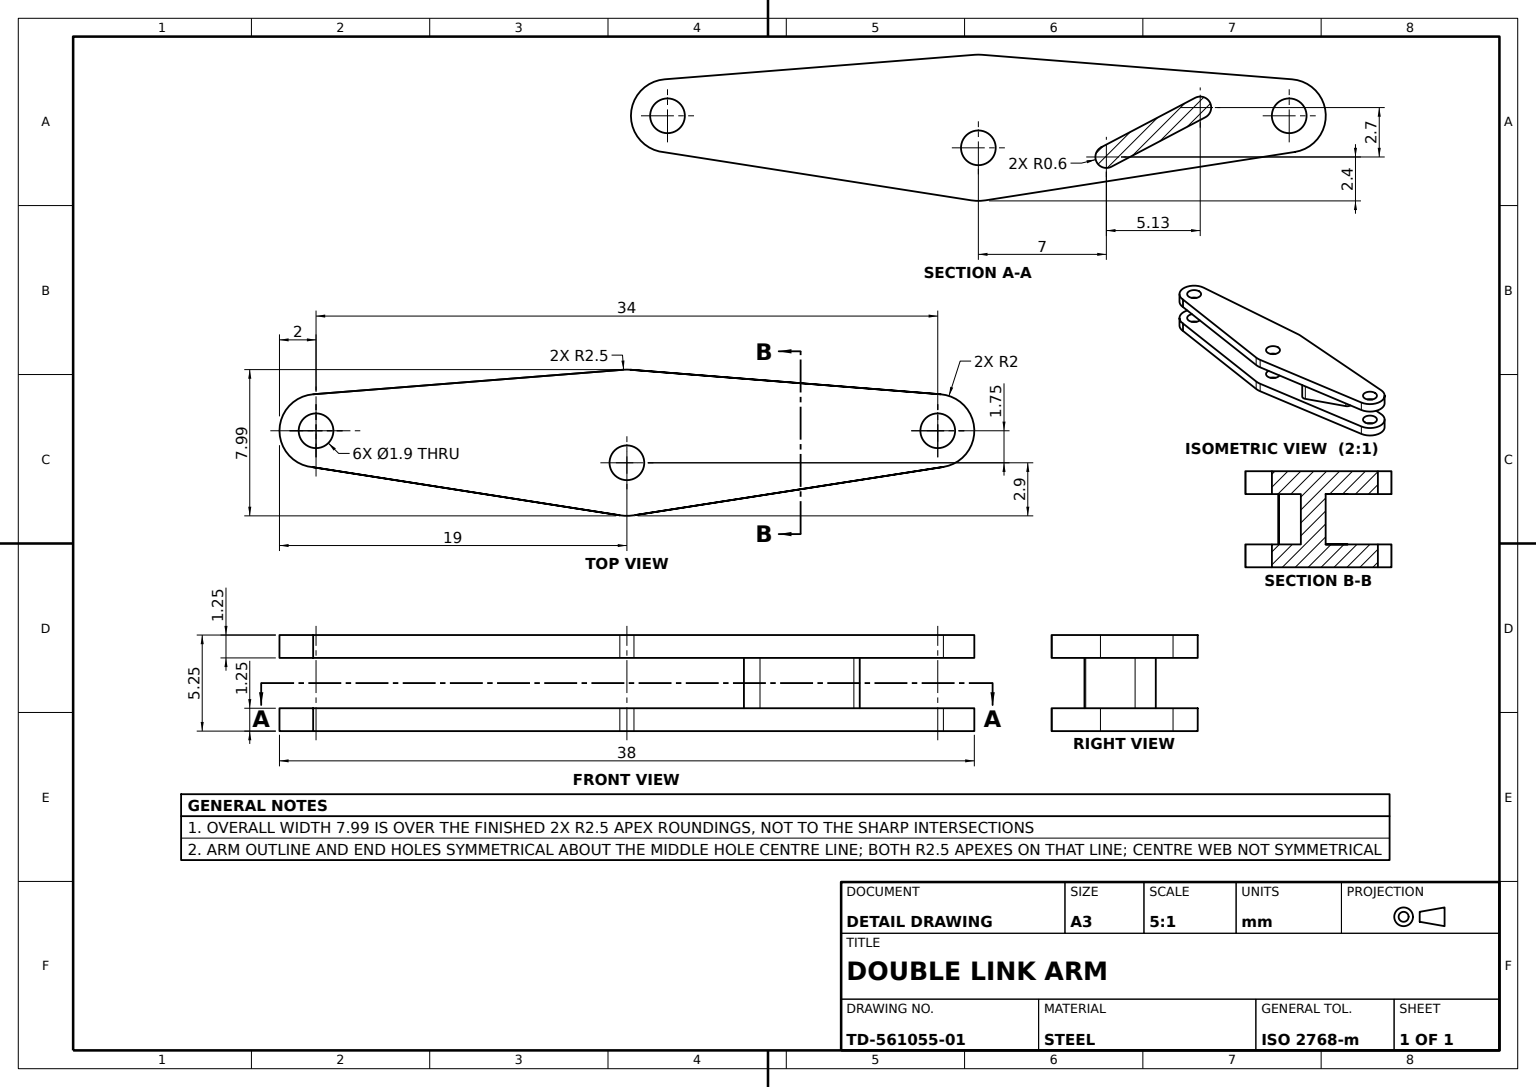
ISO-10303-21;
HEADER;
FILE_DESCRIPTION((''),'2;1');
FILE_NAME('','',(''),(''),'','','');
FILE_SCHEMA(('AUTOMOTIVE_DESIGN'));
ENDSEC;
DATA;
#1=APPLICATION_CONTEXT('');
#2=PRODUCT_CONTEXT('',#1,'mechanical');
#3=PRODUCT('','','',(#2));
#4=PRODUCT_DEFINITION_FORMATION('','',#3);
#5=PRODUCT_DEFINITION_CONTEXT('',#1,'design');
#6=PRODUCT_DEFINITION('','',#4,#5);
#7=PRODUCT_DEFINITION_SHAPE('','',#6);
#8=(LENGTH_UNIT()NAMED_UNIT(*)SI_UNIT(.MILLI.,.METRE.));
#9=(NAMED_UNIT(*)PLANE_ANGLE_UNIT()SI_UNIT($,.RADIAN.));
#10=(NAMED_UNIT(*)SI_UNIT($,.STERADIAN.)SOLID_ANGLE_UNIT());
#11=UNCERTAINTY_MEASURE_WITH_UNIT(LENGTH_MEASURE(1.E-05),#8,'distance_accuracy_value','');
#12=(GEOMETRIC_REPRESENTATION_CONTEXT(3)GLOBAL_UNCERTAINTY_ASSIGNED_CONTEXT((#11))GLOBAL_UNIT_ASSIGNED_CONTEXT((#8,#9,#10))REPRESENTATION_CONTEXT('',''));
#13=CARTESIAN_POINT('',(7.,-1.375,2.85));
#14=VERTEX_POINT('',#13);
#15=CARTESIAN_POINT('',(7.,1.375,2.85));
#16=VERTEX_POINT('',#15);
#17=CARTESIAN_POINT('',(7.,-2.627,2.85));
#18=DIRECTION('',(0.,1.,0.));
#19=VECTOR('',#18,1000.);
#20=LINE('',#17,#19);
#21=EDGE_CURVE('',#14,#16,#20,.T.);
#22=ORIENTED_EDGE('',*,*,#21,.F.);
#23=CARTESIAN_POINT('',(7.27931,-1.375,2.781023));
#24=VERTEX_POINT('',#23);
#25=CARTESIAN_POINT('',(7.,-1.375,2.25));
#26=DIRECTION('',(0.,0.,-1.));
#27=AXIS2_PLACEMENT_3D('',#25,#18,#26);
#28=CIRCLE('',#27,0.6);
#29=EDGE_CURVE('',#14,#24,#28,.T.);
#30=ORIENTED_EDGE('',*,*,#29,.T.);
#31=CARTESIAN_POINT('',(7.27931,1.375,2.781023));
#32=VERTEX_POINT('',#31);
#33=CARTESIAN_POINT('',(7.27931,-2.627,2.781023));
#34=LINE('',#33,#19);
#35=EDGE_CURVE('',#24,#32,#34,.T.);
#36=ORIENTED_EDGE('',*,*,#35,.T.);
#37=CARTESIAN_POINT('',(7.,1.375,2.25));
#38=DIRECTION('',(0.,0.,1.));
#39=AXIS2_PLACEMENT_3D('',#37,#18,#38);
#40=CIRCLE('',#39,0.6);
#41=EDGE_CURVE('',#16,#32,#40,.T.);
#42=ORIENTED_EDGE('',*,*,#41,.F.);
#43=EDGE_LOOP('',(#22,#30,#36,#42));
#44=FACE_OUTER_BOUND('',#43,.T.);
#45=CARTESIAN_POINT('',(7.,-2.627,2.25));
#46=AXIS2_PLACEMENT_3D('',#45,#18,#38);
#47=CYLINDRICAL_SURFACE('',#46,0.6);
#48=ADVANCED_FACE('',(#44),#47,.T.);
#49=CARTESIAN_POINT('',(-17.,-2.625,-0.95));
#50=VERTEX_POINT('',#49);
#51=CARTESIAN_POINT('',(-17.,-2.625,0.95));
#52=VERTEX_POINT('',#51);
#53=CARTESIAN_POINT('',(-17.,-2.625,0.));
#54=AXIS2_PLACEMENT_3D('',#53,#18,#38);
#55=CIRCLE('',#54,0.95);
#56=EDGE_CURVE('',#50,#52,#55,.T.);
#57=ORIENTED_EDGE('',*,*,#56,.F.);
#58=CARTESIAN_POINT('',(-17.,-1.375,-0.95));
#59=VERTEX_POINT('',#58);
#60=CARTESIAN_POINT('',(-17.,2.625,-0.95));
#61=DIRECTION('',(0.,-1.,0.));
#62=VECTOR('',#61,1000.);
#63=LINE('',#60,#62);
#64=EDGE_CURVE('',#59,#50,#63,.T.);
#65=ORIENTED_EDGE('',*,*,#64,.F.);
#66=CARTESIAN_POINT('',(-17.,-1.375,0.95));
#67=VERTEX_POINT('',#66);
#68=CARTESIAN_POINT('',(-17.,-1.375,0.));
#69=AXIS2_PLACEMENT_3D('',#68,#61,#26);
#70=CIRCLE('',#69,0.95);
#71=EDGE_CURVE('',#67,#59,#70,.T.);
#72=ORIENTED_EDGE('',*,*,#71,.F.);
#73=CARTESIAN_POINT('',(-17.,2.625,0.95));
#74=LINE('',#73,#62);
#75=EDGE_CURVE('',#67,#52,#74,.T.);
#76=ORIENTED_EDGE('',*,*,#75,.T.);
#77=EDGE_LOOP('',(#57,#65,#72,#76));
#78=FACE_OUTER_BOUND('',#77,.T.);
#79=CARTESIAN_POINT('',(-17.,2.625,0.));
#80=AXIS2_PLACEMENT_3D('',#79,#61,#26);
#81=CYLINDRICAL_SURFACE('',#80,0.95);
#82=ADVANCED_FACE('',(#78),#81,.F.);
#83=CARTESIAN_POINT('',(17.,2.625,-0.95));
#84=VERTEX_POINT('',#83);
#85=CARTESIAN_POINT('',(17.,1.375,-0.95));
#86=VERTEX_POINT('',#85);
#87=LINE('',#83,#62);
#88=EDGE_CURVE('',#84,#86,#87,.T.);
#89=ORIENTED_EDGE('',*,*,#88,.T.);
#90=CARTESIAN_POINT('',(17.,1.375,0.95));
#91=VERTEX_POINT('',#90);
#92=CARTESIAN_POINT('',(17.,1.375,0.));
#93=AXIS2_PLACEMENT_3D('',#92,#18,#38);
#94=CIRCLE('',#93,0.95);
#95=EDGE_CURVE('',#91,#86,#94,.T.);
#96=ORIENTED_EDGE('',*,*,#95,.F.);
#97=CARTESIAN_POINT('',(17.,2.625,0.95));
#98=VERTEX_POINT('',#97);
#99=LINE('',#97,#62);
#100=EDGE_CURVE('',#98,#91,#99,.T.);
#101=ORIENTED_EDGE('',*,*,#100,.F.);
#102=CARTESIAN_POINT('',(17.,2.625,0.));
#103=AXIS2_PLACEMENT_3D('',#102,#18,#38);
#104=CIRCLE('',#103,0.95);
#105=EDGE_CURVE('',#98,#84,#104,.T.);
#106=ORIENTED_EDGE('',*,*,#105,.T.);
#107=EDGE_LOOP('',(#89,#96,#101,#106));
#108=FACE_OUTER_BOUND('',#107,.T.);
#109=AXIS2_PLACEMENT_3D('',#102,#61,#26);
#110=CYLINDRICAL_SURFACE('',#109,0.95);
#111=ADVANCED_FACE('',(#108),#110,.F.);
#112=CARTESIAN_POINT('',(17.157598,2.625,-1.993781));
#113=VERTEX_POINT('',#112);
#114=CARTESIAN_POINT('',(17.157598,1.375,-1.993781));
#115=VERTEX_POINT('',#114);
#116=LINE('',#112,#62);
#117=EDGE_CURVE('',#113,#115,#116,.T.);
#118=ORIENTED_EDGE('',*,*,#117,.F.);
#119=CARTESIAN_POINT('',(17.30874,2.625,1.976026));
#120=VERTEX_POINT('',#119);
#121=CIRCLE('',#103,2.);
#122=EDGE_CURVE('',#120,#113,#121,.T.);
#123=ORIENTED_EDGE('',*,*,#122,.F.);
#124=CARTESIAN_POINT('',(17.30874,1.375,1.976026));
#125=VERTEX_POINT('',#124);
#126=LINE('',#119,#62);
#127=EDGE_CURVE('',#120,#125,#126,.T.);
#128=ORIENTED_EDGE('',*,*,#127,.T.);
#129=CIRCLE('',#93,2.);
#130=EDGE_CURVE('',#125,#115,#129,.T.);
#131=ORIENTED_EDGE('',*,*,#130,.T.);
#132=EDGE_LOOP('',(#118,#123,#128,#131));
#133=FACE_OUTER_BOUND('',#132,.T.);
#134=CYLINDRICAL_SURFACE('',#109,2.);
#135=ADVANCED_FACE('',(#133),#134,.T.);
#136=CARTESIAN_POINT('',(-17.157598,2.625,1.993781));
#137=VERTEX_POINT('',#136);
#138=CARTESIAN_POINT('',(-17.157598,1.375,1.993781));
#139=VERTEX_POINT('',#138);
#140=LINE('',#136,#62);
#141=EDGE_CURVE('',#137,#139,#140,.T.);
#142=ORIENTED_EDGE('',*,*,#141,.T.);
#143=CARTESIAN_POINT('',(-0.386332,1.375,4.619904));
#144=VERTEX_POINT('',#143);
#145=DIRECTION('',(0.987961552,0.,0.154699618));
#146=VECTOR('',#145,1000.);
#147=LINE('',#138,#146);
#148=EDGE_CURVE('',#139,#144,#147,.T.);
#149=ORIENTED_EDGE('',*,*,#148,.T.);
#150=CARTESIAN_POINT('',(-0.386332,2.625,4.619904));
#151=VERTEX_POINT('',#150);
#152=LINE('',#150,#62);
#153=EDGE_CURVE('',#151,#144,#152,.T.);
#154=ORIENTED_EDGE('',*,*,#153,.F.);
#155=LINE('',#136,#146);
#156=EDGE_CURVE('',#137,#151,#155,.T.);
#157=ORIENTED_EDGE('',*,*,#156,.F.);
#158=EDGE_LOOP('',(#142,#149,#154,#157));
#159=FACE_OUTER_BOUND('',#158,.T.);
#160=DIRECTION('',(0.154699618,0.,-0.987961552));
#161=DIRECTION('',(-0.987961552,0.,-0.154699618));
#162=AXIS2_PLACEMENT_3D('',#136,#160,#161);
#163=PLANE('',#162);
#164=ADVANCED_FACE('',(#159),#163,.F.);
#165=ORIENTED_EDGE('',*,*,#156,.T.);
#166=CARTESIAN_POINT('',(0.386342,2.625,4.620033));
#167=VERTEX_POINT('',#166);
#168=CARTESIAN_POINT('',(0.000417,2.625,2.15));
#169=AXIS2_PLACEMENT_3D('',#168,#18,#38);
#170=CIRCLE('',#169,2.5);
#171=EDGE_CURVE('',#151,#167,#170,.T.);
#172=ORIENTED_EDGE('',*,*,#171,.T.);
#173=DIRECTION('',(0.988013086,0.,-0.154370148));
#174=VECTOR('',#173,1000.);
#175=LINE('',#166,#174);
#176=EDGE_CURVE('',#167,#120,#175,.T.);
#177=ORIENTED_EDGE('',*,*,#176,.T.);
#178=ORIENTED_EDGE('',*,*,#122,.T.);
#179=CARTESIAN_POINT('',(0.196998,2.625,-3.334428));
#180=VERTEX_POINT('',#179);
#181=DIRECTION('',(-0.996890523,0.,-0.078799015));
#182=VECTOR('',#181,1000.);
#183=LINE('',#179,#182);
#184=EDGE_CURVE('',#113,#180,#183,.T.);
#185=ORIENTED_EDGE('',*,*,#184,.T.);
#186=CARTESIAN_POINT('',(0.,2.625,-3.342202));
#187=VERTEX_POINT('',#186);
#188=CARTESIAN_POINT('',(0.,2.625,-0.842202));
#189=AXIS2_PLACEMENT_3D('',#188,#18,#38);
#190=CIRCLE('',#189,2.5);
#191=EDGE_CURVE('',#180,#187,#190,.T.);
#192=ORIENTED_EDGE('',*,*,#191,.T.);
#193=CARTESIAN_POINT('',(-0.196998,2.625,-3.334428));
#194=VERTEX_POINT('',#193);
#195=EDGE_CURVE('',#187,#194,#190,.T.);
#196=ORIENTED_EDGE('',*,*,#195,.T.);
#197=CARTESIAN_POINT('',(-17.157598,2.625,-1.993781));
#198=VERTEX_POINT('',#197);
#199=DIRECTION('',(-0.996890523,0.,0.078799015));
#200=VECTOR('',#199,1000.);
#201=LINE('',#197,#200);
#202=EDGE_CURVE('',#194,#198,#201,.T.);
#203=ORIENTED_EDGE('',*,*,#202,.T.);
#204=AXIS2_PLACEMENT_3D('',#79,#18,#38);
#205=CIRCLE('',#204,2.);
#206=EDGE_CURVE('',#198,#137,#205,.T.);
#207=ORIENTED_EDGE('',*,*,#206,.T.);
#208=EDGE_LOOP('',(#165,#172,#177,#178,#185,#192,#196,#203,#207));
#209=FACE_OUTER_BOUND('',#208,.T.);
#210=ORIENTED_EDGE('',*,*,#105,.F.);
#211=EDGE_CURVE('',#84,#98,#104,.T.);
#212=ORIENTED_EDGE('',*,*,#211,.F.);
#213=EDGE_LOOP('',(#210,#212));
#214=FACE_BOUND('',#213,.T.);
#215=VERTEX_POINT('',#73);
#216=VERTEX_POINT('',#60);
#217=CIRCLE('',#204,0.95);
#218=EDGE_CURVE('',#215,#216,#217,.T.);
#219=ORIENTED_EDGE('',*,*,#218,.F.);
#220=EDGE_CURVE('',#216,#215,#217,.T.);
#221=ORIENTED_EDGE('',*,*,#220,.F.);
#222=EDGE_LOOP('',(#219,#221));
#223=FACE_BOUND('',#222,.T.);
#224=CARTESIAN_POINT('',(0.,2.625,0.8));
#225=VERTEX_POINT('',#224);
#226=CARTESIAN_POINT('',(0.,2.625,2.7));
#227=VERTEX_POINT('',#226);
#228=CARTESIAN_POINT('',(0.,2.625,1.75));
#229=AXIS2_PLACEMENT_3D('',#228,#18,#38);
#230=CIRCLE('',#229,0.95);
#231=EDGE_CURVE('',#225,#227,#230,.T.);
#232=ORIENTED_EDGE('',*,*,#231,.F.);
#233=EDGE_CURVE('',#227,#225,#230,.T.);
#234=ORIENTED_EDGE('',*,*,#233,.F.);
#235=EDGE_LOOP('',(#232,#234));
#236=FACE_BOUND('',#235,.T.);
#237=PLANE('',#169);
#238=ADVANCED_FACE('',(#209,#214,#223,#236),#237,.T.);
#239=CARTESIAN_POINT('',(11.853915,-1.375,-0.981023));
#240=VERTEX_POINT('',#239);
#241=CARTESIAN_POINT('',(11.853915,1.375,-0.981023));
#242=VERTEX_POINT('',#241);
#243=CARTESIAN_POINT('',(11.853915,-2.627,-0.981023));
#244=LINE('',#243,#19);
#245=EDGE_CURVE('',#240,#242,#244,.T.);
#246=ORIENTED_EDGE('',*,*,#245,.T.);
#247=CARTESIAN_POINT('',(12.412535,1.375,0.081023));
#248=VERTEX_POINT('',#247);
#249=CARTESIAN_POINT('',(12.133225,1.375,-0.45));
#250=AXIS2_PLACEMENT_3D('',#249,#18,#38);
#251=CIRCLE('',#250,0.6);
#252=EDGE_CURVE('',#248,#242,#251,.T.);
#253=ORIENTED_EDGE('',*,*,#252,.F.);
#254=CARTESIAN_POINT('',(12.412535,-1.375,0.081023));
#255=VERTEX_POINT('',#254);
#256=CARTESIAN_POINT('',(12.412535,-2.627,0.081023));
#257=LINE('',#256,#19);
#258=EDGE_CURVE('',#255,#248,#257,.T.);
#259=ORIENTED_EDGE('',*,*,#258,.F.);
#260=CARTESIAN_POINT('',(12.133225,-1.375,-0.45));
#261=AXIS2_PLACEMENT_3D('',#260,#18,#26);
#262=CIRCLE('',#261,0.6);
#263=EDGE_CURVE('',#255,#240,#262,.T.);
#264=ORIENTED_EDGE('',*,*,#263,.T.);
#265=EDGE_LOOP('',(#246,#253,#259,#264));
#266=FACE_OUTER_BOUND('',#265,.T.);
#267=CARTESIAN_POINT('',(12.133225,-2.627,-0.45));
#268=AXIS2_PLACEMENT_3D('',#267,#18,#38);
#269=CYLINDRICAL_SURFACE('',#268,0.6);
#270=ADVANCED_FACE('',(#266),#269,.T.);
#271=CARTESIAN_POINT('',(0.386342,-1.375,4.620033));
#272=VERTEX_POINT('',#271);
#273=CARTESIAN_POINT('',(0.386342,-2.625,4.620033));
#274=VERTEX_POINT('',#273);
#275=LINE('',#166,#62);
#276=EDGE_CURVE('',#272,#274,#275,.T.);
#277=ORIENTED_EDGE('',*,*,#276,.T.);
#278=CARTESIAN_POINT('',(17.30874,-2.625,1.976026));
#279=VERTEX_POINT('',#278);
#280=LINE('',#273,#174);
#281=EDGE_CURVE('',#274,#279,#280,.T.);
#282=ORIENTED_EDGE('',*,*,#281,.T.);
#283=CARTESIAN_POINT('',(17.30874,-1.375,1.976026));
#284=VERTEX_POINT('',#283);
#285=EDGE_CURVE('',#284,#279,#126,.T.);
#286=ORIENTED_EDGE('',*,*,#285,.F.);
#287=DIRECTION('',(-0.988013086,0.,0.154370148));
#288=VECTOR('',#287,1000.);
#289=LINE('',#271,#288);
#290=EDGE_CURVE('',#284,#272,#289,.T.);
#291=ORIENTED_EDGE('',*,*,#290,.T.);
#292=EDGE_LOOP('',(#277,#282,#286,#291));
#293=FACE_OUTER_BOUND('',#292,.T.);
#294=DIRECTION('',(-0.154370148,0.,-0.988013086));
#295=AXIS2_PLACEMENT_3D('',#166,#294,#287);
#296=PLANE('',#295);
#297=ADVANCED_FACE('',(#293),#296,.F.);
#298=CARTESIAN_POINT('',(0.,1.375,2.7));
#299=VERTEX_POINT('',#298);
#300=LINE('',#226,#62);
#301=EDGE_CURVE('',#227,#299,#300,.T.);
#302=ORIENTED_EDGE('',*,*,#301,.T.);
#303=CARTESIAN_POINT('',(0.,1.375,0.8));
#304=VERTEX_POINT('',#303);
#305=CARTESIAN_POINT('',(0.,1.375,1.75));
#306=AXIS2_PLACEMENT_3D('',#305,#18,#38);
#307=CIRCLE('',#306,0.95);
#308=EDGE_CURVE('',#304,#299,#307,.T.);
#309=ORIENTED_EDGE('',*,*,#308,.F.);
#310=LINE('',#224,#62);
#311=EDGE_CURVE('',#225,#304,#310,.T.);
#312=ORIENTED_EDGE('',*,*,#311,.F.);
#313=ORIENTED_EDGE('',*,*,#231,.T.);
#314=EDGE_LOOP('',(#302,#309,#312,#313));
#315=FACE_OUTER_BOUND('',#314,.T.);
#316=AXIS2_PLACEMENT_3D('',#228,#61,#26);
#317=CYLINDRICAL_SURFACE('',#316,0.95);
#318=ADVANCED_FACE('',(#315),#317,.F.);
#319=EDGE_CURVE('',#59,#67,#70,.T.);
#320=ORIENTED_EDGE('',*,*,#319,.T.);
#321=ORIENTED_EDGE('',*,*,#71,.T.);
#322=EDGE_LOOP('',(#320,#321));
#323=FACE_BOUND('',#322,.T.);
#324=CARTESIAN_POINT('',(17.,-1.375,0.95));
#325=VERTEX_POINT('',#324);
#326=CARTESIAN_POINT('',(17.,-1.375,-0.95));
#327=VERTEX_POINT('',#326);
#328=CARTESIAN_POINT('',(17.,-1.375,0.));
#329=AXIS2_PLACEMENT_3D('',#328,#61,#26);
#330=CIRCLE('',#329,0.95);
#331=EDGE_CURVE('',#325,#327,#330,.T.);
#332=ORIENTED_EDGE('',*,*,#331,.T.);
#333=EDGE_CURVE('',#327,#325,#330,.T.);
#334=ORIENTED_EDGE('',*,*,#333,.T.);
#335=EDGE_LOOP('',(#332,#334));
#336=FACE_BOUND('',#335,.T.);
#337=CARTESIAN_POINT('',(-0.196998,-1.375,-3.334428));
#338=VERTEX_POINT('',#337);
#339=CARTESIAN_POINT('',(0.,-1.375,-3.342202));
#340=VERTEX_POINT('',#339);
#341=CARTESIAN_POINT('',(0.,-1.375,-0.842202));
#342=AXIS2_PLACEMENT_3D('',#341,#61,#26);
#343=CIRCLE('',#342,2.5);
#344=EDGE_CURVE('',#338,#340,#343,.T.);
#345=ORIENTED_EDGE('',*,*,#344,.F.);
#346=CARTESIAN_POINT('',(-17.157598,-1.375,-1.993781));
#347=VERTEX_POINT('',#346);
#348=DIRECTION('',(0.996890523,0.,-0.078799015));
#349=VECTOR('',#348,1000.);
#350=LINE('',#346,#349);
#351=EDGE_CURVE('',#347,#338,#350,.T.);
#352=ORIENTED_EDGE('',*,*,#351,.F.);
#353=CARTESIAN_POINT('',(-17.157598,-1.375,1.993781));
#354=VERTEX_POINT('',#353);
#355=CIRCLE('',#69,2.);
#356=EDGE_CURVE('',#354,#347,#355,.T.);
#357=ORIENTED_EDGE('',*,*,#356,.F.);
#358=CARTESIAN_POINT('',(-0.386332,-1.375,4.619904));
#359=VERTEX_POINT('',#358);
#360=VECTOR('',#161,1000.);
#361=LINE('',#353,#360);
#362=EDGE_CURVE('',#359,#354,#361,.T.);
#363=ORIENTED_EDGE('',*,*,#362,.F.);
#364=CARTESIAN_POINT('',(0.000417,-1.375,2.15));
#365=AXIS2_PLACEMENT_3D('',#364,#61,#26);
#366=CIRCLE('',#365,2.5);
#367=EDGE_CURVE('',#272,#359,#366,.T.);
#368=ORIENTED_EDGE('',*,*,#367,.F.);
#369=ORIENTED_EDGE('',*,*,#290,.F.);
#370=CARTESIAN_POINT('',(17.157598,-1.375,-1.993781));
#371=VERTEX_POINT('',#370);
#372=CIRCLE('',#329,2.);
#373=EDGE_CURVE('',#371,#284,#372,.T.);
#374=ORIENTED_EDGE('',*,*,#373,.F.);
#375=CARTESIAN_POINT('',(0.196998,-1.375,-3.334428));
#376=VERTEX_POINT('',#375);
#377=DIRECTION('',(0.996890523,0.,0.078799015));
#378=VECTOR('',#377,1000.);
#379=LINE('',#375,#378);
#380=EDGE_CURVE('',#376,#371,#379,.T.);
#381=ORIENTED_EDGE('',*,*,#380,.F.);
#382=EDGE_CURVE('',#340,#376,#343,.T.);
#383=ORIENTED_EDGE('',*,*,#382,.F.);
#384=EDGE_LOOP('',(#345,#352,#357,#363,#368,#369,#374,#381,#383));
#385=FACE_OUTER_BOUND('',#384,.T.);
#386=DIRECTION('',(0.885038812,0.,-0.465517241));
#387=VECTOR('',#386,1000.);
#388=LINE('',#23,#387);
#389=EDGE_CURVE('',#24,#255,#388,.T.);
#390=ORIENTED_EDGE('',*,*,#389,.F.);
#391=ORIENTED_EDGE('',*,*,#29,.F.);
#392=CARTESIAN_POINT('',(6.72069,-1.375,1.718977));
#393=VERTEX_POINT('',#392);
#394=EDGE_CURVE('',#393,#14,#28,.T.);
#395=ORIENTED_EDGE('',*,*,#394,.F.);
#396=DIRECTION('',(-0.885038812,0.,0.465517241));
#397=VECTOR('',#396,1000.);
#398=LINE('',#392,#397);
#399=EDGE_CURVE('',#240,#393,#398,.T.);
#400=ORIENTED_EDGE('',*,*,#399,.F.);
#401=ORIENTED_EDGE('',*,*,#263,.F.);
#402=EDGE_LOOP('',(#390,#391,#395,#400,#401));
#403=FACE_BOUND('',#402,.T.);
#404=CARTESIAN_POINT('',(0.,-1.375,2.7));
#405=VERTEX_POINT('',#404);
#406=CARTESIAN_POINT('',(0.,-1.375,0.8));
#407=VERTEX_POINT('',#406);
#408=CARTESIAN_POINT('',(0.,-1.375,1.75));
#409=AXIS2_PLACEMENT_3D('',#408,#61,#26);
#410=CIRCLE('',#409,0.95);
#411=EDGE_CURVE('',#405,#407,#410,.T.);
#412=ORIENTED_EDGE('',*,*,#411,.T.);
#413=EDGE_CURVE('',#407,#405,#410,.T.);
#414=ORIENTED_EDGE('',*,*,#413,.T.);
#415=EDGE_LOOP('',(#412,#414));
#416=FACE_BOUND('',#415,.T.);
#417=CARTESIAN_POINT('',(-19.564242,-1.375,-22.625));
#418=AXIS2_PLACEMENT_3D('',#417,#61,#26);
#419=PLANE('',#418);
#420=ADVANCED_FACE('',(#323,#336,#385,#403,#416),#419,.F.);
#421=ORIENTED_EDGE('',*,*,#258,.T.);
#422=LINE('',#31,#387);
#423=EDGE_CURVE('',#32,#248,#422,.T.);
#424=ORIENTED_EDGE('',*,*,#423,.F.);
#425=ORIENTED_EDGE('',*,*,#35,.F.);
#426=ORIENTED_EDGE('',*,*,#389,.T.);
#427=EDGE_LOOP('',(#421,#424,#425,#426));
#428=FACE_OUTER_BOUND('',#427,.T.);
#429=DIRECTION('',(0.465517241,0.,0.885038812));
#430=AXIS2_PLACEMENT_3D('',#33,#429,#386);
#431=PLANE('',#430);
#432=ADVANCED_FACE('',(#428),#431,.T.);
#433=ORIENTED_EDGE('',*,*,#380,.T.);
#434=CARTESIAN_POINT('',(17.157598,-2.625,-1.993781));
#435=VERTEX_POINT('',#434);
#436=EDGE_CURVE('',#371,#435,#116,.T.);
#437=ORIENTED_EDGE('',*,*,#436,.T.);
#438=CARTESIAN_POINT('',(0.196998,-2.625,-3.334428));
#439=VERTEX_POINT('',#438);
#440=LINE('',#438,#182);
#441=EDGE_CURVE('',#435,#439,#440,.T.);
#442=ORIENTED_EDGE('',*,*,#441,.T.);
#443=LINE('',#179,#62);
#444=EDGE_CURVE('',#376,#439,#443,.T.);
#445=ORIENTED_EDGE('',*,*,#444,.F.);
#446=EDGE_LOOP('',(#433,#437,#442,#445));
#447=FACE_OUTER_BOUND('',#446,.T.);
#448=DIRECTION('',(-0.078799015,0.,0.996890523));
#449=AXIS2_PLACEMENT_3D('',#179,#448,#377);
#450=PLANE('',#449);
#451=ADVANCED_FACE('',(#447),#450,.F.);
#452=ORIENTED_EDGE('',*,*,#276,.F.);
#453=ORIENTED_EDGE('',*,*,#367,.T.);
#454=CARTESIAN_POINT('',(-0.386332,-2.625,4.619904));
#455=VERTEX_POINT('',#454);
#456=EDGE_CURVE('',#359,#455,#152,.T.);
#457=ORIENTED_EDGE('',*,*,#456,.T.);
#458=CARTESIAN_POINT('',(0.000417,-2.625,2.15));
#459=AXIS2_PLACEMENT_3D('',#458,#18,#38);
#460=CIRCLE('',#459,2.5);
#461=EDGE_CURVE('',#455,#274,#460,.T.);
#462=ORIENTED_EDGE('',*,*,#461,.T.);
#463=EDGE_LOOP('',(#452,#453,#457,#462));
#464=FACE_OUTER_BOUND('',#463,.T.);
#465=AXIS2_PLACEMENT_3D('',#168,#61,#26);
#466=CYLINDRICAL_SURFACE('',#465,2.5);
#467=ADVANCED_FACE('',(#464),#466,.T.);
#468=CARTESIAN_POINT('',(6.72069,1.375,1.718977));
#469=VERTEX_POINT('',#468);
#470=CARTESIAN_POINT('',(6.72069,-2.627,1.718977));
#471=LINE('',#470,#19);
#472=EDGE_CURVE('',#393,#469,#471,.T.);
#473=ORIENTED_EDGE('',*,*,#472,.T.);
#474=LINE('',#468,#397);
#475=EDGE_CURVE('',#242,#469,#474,.T.);
#476=ORIENTED_EDGE('',*,*,#475,.F.);
#477=ORIENTED_EDGE('',*,*,#245,.F.);
#478=ORIENTED_EDGE('',*,*,#399,.T.);
#479=EDGE_LOOP('',(#473,#476,#477,#478));
#480=FACE_OUTER_BOUND('',#479,.T.);
#481=DIRECTION('',(-0.465517241,0.,-0.885038812));
#482=AXIS2_PLACEMENT_3D('',#470,#481,#396);
#483=PLANE('',#482);
#484=ADVANCED_FACE('',(#480),#483,.T.);
#485=ORIENTED_EDGE('',*,*,#344,.T.);
#486=CARTESIAN_POINT('',(0.,-2.625,-3.342202));
#487=VERTEX_POINT('',#486);
#488=LINE('',#186,#62);
#489=EDGE_CURVE('',#340,#487,#488,.T.);
#490=ORIENTED_EDGE('',*,*,#489,.T.);
#491=CARTESIAN_POINT('',(-0.196998,-2.625,-3.334428));
#492=VERTEX_POINT('',#491);
#493=CARTESIAN_POINT('',(0.,-2.625,-0.842202));
#494=AXIS2_PLACEMENT_3D('',#493,#18,#38);
#495=CIRCLE('',#494,2.5);
#496=EDGE_CURVE('',#487,#492,#495,.T.);
#497=ORIENTED_EDGE('',*,*,#496,.T.);
#498=LINE('',#193,#62);
#499=EDGE_CURVE('',#338,#492,#498,.T.);
#500=ORIENTED_EDGE('',*,*,#499,.F.);
#501=EDGE_LOOP('',(#485,#490,#497,#500));
#502=FACE_OUTER_BOUND('',#501,.T.);
#503=AXIS2_PLACEMENT_3D('',#188,#61,#26);
#504=CYLINDRICAL_SURFACE('',#503,2.5);
#505=ADVANCED_FACE('',(#502),#504,.T.);
#506=CARTESIAN_POINT('',(-17.157598,-2.625,1.993781));
#507=VERTEX_POINT('',#506);
#508=EDGE_CURVE('',#354,#507,#140,.T.);
#509=ORIENTED_EDGE('',*,*,#508,.T.);
#510=LINE('',#506,#146);
#511=EDGE_CURVE('',#507,#455,#510,.T.);
#512=ORIENTED_EDGE('',*,*,#511,.T.);
#513=ORIENTED_EDGE('',*,*,#456,.F.);
#514=ORIENTED_EDGE('',*,*,#362,.T.);
#515=EDGE_LOOP('',(#509,#512,#513,#514));
#516=FACE_OUTER_BOUND('',#515,.T.);
#517=ADVANCED_FACE('',(#516),#163,.F.);
#518=ORIENTED_EDGE('',*,*,#331,.F.);
#519=CARTESIAN_POINT('',(17.,-2.625,0.95));
#520=VERTEX_POINT('',#519);
#521=EDGE_CURVE('',#325,#520,#99,.T.);
#522=ORIENTED_EDGE('',*,*,#521,.T.);
#523=CARTESIAN_POINT('',(17.,-2.625,-0.95));
#524=VERTEX_POINT('',#523);
#525=CARTESIAN_POINT('',(17.,-2.625,0.));
#526=AXIS2_PLACEMENT_3D('',#525,#18,#38);
#527=CIRCLE('',#526,0.95);
#528=EDGE_CURVE('',#524,#520,#527,.T.);
#529=ORIENTED_EDGE('',*,*,#528,.F.);
#530=EDGE_CURVE('',#327,#524,#87,.T.);
#531=ORIENTED_EDGE('',*,*,#530,.F.);
#532=EDGE_LOOP('',(#518,#522,#529,#531));
#533=FACE_OUTER_BOUND('',#532,.T.);
#534=ADVANCED_FACE('',(#533),#110,.F.);
#535=ORIENTED_EDGE('',*,*,#301,.F.);
#536=ORIENTED_EDGE('',*,*,#233,.T.);
#537=ORIENTED_EDGE('',*,*,#311,.T.);
#538=EDGE_CURVE('',#299,#304,#307,.T.);
#539=ORIENTED_EDGE('',*,*,#538,.F.);
#540=EDGE_LOOP('',(#535,#536,#537,#539));
#541=FACE_OUTER_BOUND('',#540,.T.);
#542=ADVANCED_FACE('',(#541),#317,.F.);
#543=CARTESIAN_POINT('',(-17.157598,1.375,-1.993781));
#544=VERTEX_POINT('',#543);
#545=LINE('',#197,#62);
#546=EDGE_CURVE('',#198,#544,#545,.T.);
#547=ORIENTED_EDGE('',*,*,#546,.F.);
#548=ORIENTED_EDGE('',*,*,#202,.F.);
#549=CARTESIAN_POINT('',(-0.196998,1.375,-3.334428));
#550=VERTEX_POINT('',#549);
#551=EDGE_CURVE('',#194,#550,#498,.T.);
#552=ORIENTED_EDGE('',*,*,#551,.T.);
#553=LINE('',#543,#200);
#554=EDGE_CURVE('',#550,#544,#553,.T.);
#555=ORIENTED_EDGE('',*,*,#554,.T.);
#556=EDGE_LOOP('',(#547,#548,#552,#555));
#557=FACE_OUTER_BOUND('',#556,.T.);
#558=DIRECTION('',(0.078799015,0.,0.996890523));
#559=AXIS2_PLACEMENT_3D('',#197,#558,#348);
#560=PLANE('',#559);
#561=ADVANCED_FACE('',(#557),#560,.F.);
#562=ORIENTED_EDGE('',*,*,#285,.T.);
#563=CIRCLE('',#526,2.);
#564=EDGE_CURVE('',#279,#435,#563,.T.);
#565=ORIENTED_EDGE('',*,*,#564,.T.);
#566=ORIENTED_EDGE('',*,*,#436,.F.);
#567=ORIENTED_EDGE('',*,*,#373,.T.);
#568=EDGE_LOOP('',(#562,#565,#566,#567));
#569=FACE_OUTER_BOUND('',#568,.T.);
#570=ADVANCED_FACE('',(#569),#134,.T.);
#571=CARTESIAN_POINT('',(0.,1.375,-3.342202));
#572=VERTEX_POINT('',#571);
#573=EDGE_CURVE('',#187,#572,#488,.T.);
#574=ORIENTED_EDGE('',*,*,#573,.T.);
#575=CARTESIAN_POINT('',(0.,1.375,-0.842202));
#576=AXIS2_PLACEMENT_3D('',#575,#18,#38);
#577=CIRCLE('',#576,2.5);
#578=EDGE_CURVE('',#572,#550,#577,.T.);
#579=ORIENTED_EDGE('',*,*,#578,.T.);
#580=ORIENTED_EDGE('',*,*,#551,.F.);
#581=ORIENTED_EDGE('',*,*,#195,.F.);
#582=EDGE_LOOP('',(#574,#579,#580,#581));
#583=FACE_OUTER_BOUND('',#582,.T.);
#584=ADVANCED_FACE('',(#583),#504,.T.);
#585=ORIENTED_EDGE('',*,*,#444,.T.);
#586=EDGE_CURVE('',#439,#487,#495,.T.);
#587=ORIENTED_EDGE('',*,*,#586,.T.);
#588=ORIENTED_EDGE('',*,*,#489,.F.);
#589=ORIENTED_EDGE('',*,*,#382,.T.);
#590=EDGE_LOOP('',(#585,#587,#588,#589));
#591=FACE_OUTER_BOUND('',#590,.T.);
#592=ADVANCED_FACE('',(#591),#504,.T.);
#593=ORIENTED_EDGE('',*,*,#75,.F.);
#594=ORIENTED_EDGE('',*,*,#319,.F.);
#595=ORIENTED_EDGE('',*,*,#64,.T.);
#596=EDGE_CURVE('',#52,#50,#55,.T.);
#597=ORIENTED_EDGE('',*,*,#596,.F.);
#598=EDGE_LOOP('',(#593,#594,#595,#597));
#599=FACE_OUTER_BOUND('',#598,.T.);
#600=ADVANCED_FACE('',(#599),#81,.F.);
#601=ORIENTED_EDGE('',*,*,#184,.F.);
#602=ORIENTED_EDGE('',*,*,#117,.T.);
#603=CARTESIAN_POINT('',(0.196998,1.375,-3.334428));
#604=VERTEX_POINT('',#603);
#605=LINE('',#603,#182);
#606=EDGE_CURVE('',#115,#604,#605,.T.);
#607=ORIENTED_EDGE('',*,*,#606,.T.);
#608=EDGE_CURVE('',#180,#604,#443,.T.);
#609=ORIENTED_EDGE('',*,*,#608,.F.);
#610=EDGE_LOOP('',(#601,#602,#607,#609));
#611=FACE_OUTER_BOUND('',#610,.T.);
#612=ADVANCED_FACE('',(#611),#450,.F.);
#613=CARTESIAN_POINT('',(-17.,1.375,0.95));
#614=VERTEX_POINT('',#613);
#615=EDGE_CURVE('',#215,#614,#74,.T.);
#616=ORIENTED_EDGE('',*,*,#615,.F.);
#617=ORIENTED_EDGE('',*,*,#218,.T.);
#618=CARTESIAN_POINT('',(-17.,1.375,-0.95));
#619=VERTEX_POINT('',#618);
#620=EDGE_CURVE('',#216,#619,#63,.T.);
#621=ORIENTED_EDGE('',*,*,#620,.T.);
#622=CARTESIAN_POINT('',(-17.,1.375,0.));
#623=AXIS2_PLACEMENT_3D('',#622,#18,#38);
#624=CIRCLE('',#623,0.95);
#625=EDGE_CURVE('',#614,#619,#624,.T.);
#626=ORIENTED_EDGE('',*,*,#625,.F.);
#627=EDGE_LOOP('',(#616,#617,#621,#626));
#628=FACE_OUTER_BOUND('',#627,.T.);
#629=ADVANCED_FACE('',(#628),#81,.F.);
#630=CARTESIAN_POINT('',(-17.157598,-2.625,-1.993781));
#631=VERTEX_POINT('',#630);
#632=LINE('',#630,#200);
#633=EDGE_CURVE('',#492,#631,#632,.T.);
#634=ORIENTED_EDGE('',*,*,#633,.T.);
#635=EDGE_CURVE('',#347,#631,#545,.T.);
#636=ORIENTED_EDGE('',*,*,#635,.F.);
#637=ORIENTED_EDGE('',*,*,#351,.T.);
#638=ORIENTED_EDGE('',*,*,#499,.T.);
#639=EDGE_LOOP('',(#634,#636,#637,#638));
#640=FACE_OUTER_BOUND('',#639,.T.);
#641=ADVANCED_FACE('',(#640),#560,.F.);
#642=ORIENTED_EDGE('',*,*,#521,.F.);
#643=ORIENTED_EDGE('',*,*,#333,.F.);
#644=ORIENTED_EDGE('',*,*,#530,.T.);
#645=EDGE_CURVE('',#520,#524,#527,.T.);
#646=ORIENTED_EDGE('',*,*,#645,.F.);
#647=EDGE_LOOP('',(#642,#643,#644,#646));
#648=FACE_OUTER_BOUND('',#647,.T.);
#649=ADVANCED_FACE('',(#648),#110,.F.);
#650=CARTESIAN_POINT('',(0.386342,1.375,4.620033));
#651=VERTEX_POINT('',#650);
#652=LINE('',#650,#174);
#653=EDGE_CURVE('',#651,#125,#652,.T.);
#654=ORIENTED_EDGE('',*,*,#653,.T.);
#655=ORIENTED_EDGE('',*,*,#127,.F.);
#656=ORIENTED_EDGE('',*,*,#176,.F.);
#657=EDGE_CURVE('',#167,#651,#275,.T.);
#658=ORIENTED_EDGE('',*,*,#657,.T.);
#659=EDGE_LOOP('',(#654,#655,#656,#658));
#660=FACE_OUTER_BOUND('',#659,.T.);
#661=ADVANCED_FACE('',(#660),#296,.F.);
#662=ORIENTED_EDGE('',*,*,#657,.F.);
#663=ORIENTED_EDGE('',*,*,#171,.F.);
#664=ORIENTED_EDGE('',*,*,#153,.T.);
#665=CARTESIAN_POINT('',(0.000417,1.375,2.15));
#666=AXIS2_PLACEMENT_3D('',#665,#18,#38);
#667=CIRCLE('',#666,2.5);
#668=EDGE_CURVE('',#144,#651,#667,.T.);
#669=ORIENTED_EDGE('',*,*,#668,.T.);
#670=EDGE_LOOP('',(#662,#663,#664,#669));
#671=FACE_OUTER_BOUND('',#670,.T.);
#672=ADVANCED_FACE('',(#671),#466,.T.);
#673=ORIENTED_EDGE('',*,*,#413,.F.);
#674=CARTESIAN_POINT('',(0.,-2.625,0.8));
#675=VERTEX_POINT('',#674);
#676=EDGE_CURVE('',#407,#675,#310,.T.);
#677=ORIENTED_EDGE('',*,*,#676,.T.);
#678=CARTESIAN_POINT('',(0.,-2.625,2.7));
#679=VERTEX_POINT('',#678);
#680=CARTESIAN_POINT('',(0.,-2.625,1.75));
#681=AXIS2_PLACEMENT_3D('',#680,#18,#38);
#682=CIRCLE('',#681,0.95);
#683=EDGE_CURVE('',#679,#675,#682,.T.);
#684=ORIENTED_EDGE('',*,*,#683,.F.);
#685=EDGE_CURVE('',#405,#679,#300,.T.);
#686=ORIENTED_EDGE('',*,*,#685,.F.);
#687=EDGE_LOOP('',(#673,#677,#684,#686));
#688=FACE_OUTER_BOUND('',#687,.T.);
#689=ADVANCED_FACE('',(#688),#317,.F.);
#690=ORIENTED_EDGE('',*,*,#508,.F.);
#691=ORIENTED_EDGE('',*,*,#356,.T.);
#692=ORIENTED_EDGE('',*,*,#635,.T.);
#693=CIRCLE('',#54,2.);
#694=EDGE_CURVE('',#631,#507,#693,.T.);
#695=ORIENTED_EDGE('',*,*,#694,.T.);
#696=EDGE_LOOP('',(#690,#691,#692,#695));
#697=FACE_OUTER_BOUND('',#696,.T.);
#698=CYLINDRICAL_SURFACE('',#80,2.);
#699=ADVANCED_FACE('',(#697),#698,.T.);
#700=ORIENTED_EDGE('',*,*,#88,.F.);
#701=ORIENTED_EDGE('',*,*,#211,.T.);
#702=ORIENTED_EDGE('',*,*,#100,.T.);
#703=EDGE_CURVE('',#86,#91,#94,.T.);
#704=ORIENTED_EDGE('',*,*,#703,.F.);
#705=EDGE_LOOP('',(#700,#701,#702,#704));
#706=FACE_OUTER_BOUND('',#705,.T.);
#707=ADVANCED_FACE('',(#706),#110,.F.);
#708=ORIENTED_EDGE('',*,*,#620,.F.);
#709=ORIENTED_EDGE('',*,*,#220,.T.);
#710=ORIENTED_EDGE('',*,*,#615,.T.);
#711=EDGE_CURVE('',#619,#614,#624,.T.);
#712=ORIENTED_EDGE('',*,*,#711,.F.);
#713=EDGE_LOOP('',(#708,#709,#710,#712));
#714=FACE_OUTER_BOUND('',#713,.T.);
#715=ADVANCED_FACE('',(#714),#81,.F.);
#716=CIRCLE('',#623,2.);
#717=EDGE_CURVE('',#544,#139,#716,.T.);
#718=ORIENTED_EDGE('',*,*,#717,.T.);
#719=ORIENTED_EDGE('',*,*,#141,.F.);
#720=ORIENTED_EDGE('',*,*,#206,.F.);
#721=ORIENTED_EDGE('',*,*,#546,.T.);
#722=EDGE_LOOP('',(#718,#719,#720,#721));
#723=FACE_OUTER_BOUND('',#722,.T.);
#724=ADVANCED_FACE('',(#723),#698,.T.);
#725=EDGE_CURVE('',#469,#16,#40,.T.);
#726=ORIENTED_EDGE('',*,*,#725,.F.);
#727=ORIENTED_EDGE('',*,*,#472,.F.);
#728=ORIENTED_EDGE('',*,*,#394,.T.);
#729=ORIENTED_EDGE('',*,*,#21,.T.);
#730=EDGE_LOOP('',(#726,#727,#728,#729));
#731=FACE_OUTER_BOUND('',#730,.T.);
#732=ADVANCED_FACE('',(#731),#47,.T.);
#733=ORIENTED_EDGE('',*,*,#308,.T.);
#734=ORIENTED_EDGE('',*,*,#538,.T.);
#735=EDGE_LOOP('',(#733,#734));
#736=FACE_BOUND('',#735,.T.);
#737=ORIENTED_EDGE('',*,*,#95,.T.);
#738=ORIENTED_EDGE('',*,*,#703,.T.);
#739=EDGE_LOOP('',(#737,#738));
#740=FACE_BOUND('',#739,.T.);
#741=ORIENTED_EDGE('',*,*,#625,.T.);
#742=ORIENTED_EDGE('',*,*,#711,.T.);
#743=EDGE_LOOP('',(#741,#742));
#744=FACE_BOUND('',#743,.T.);
#745=ORIENTED_EDGE('',*,*,#252,.T.);
#746=ORIENTED_EDGE('',*,*,#475,.T.);
#747=ORIENTED_EDGE('',*,*,#725,.T.);
#748=ORIENTED_EDGE('',*,*,#41,.T.);
#749=ORIENTED_EDGE('',*,*,#423,.T.);
#750=EDGE_LOOP('',(#745,#746,#747,#748,#749));
#751=FACE_BOUND('',#750,.T.);
#752=ORIENTED_EDGE('',*,*,#717,.F.);
#753=ORIENTED_EDGE('',*,*,#554,.F.);
#754=ORIENTED_EDGE('',*,*,#578,.F.);
#755=EDGE_CURVE('',#604,#572,#577,.T.);
#756=ORIENTED_EDGE('',*,*,#755,.F.);
#757=ORIENTED_EDGE('',*,*,#606,.F.);
#758=ORIENTED_EDGE('',*,*,#130,.F.);
#759=ORIENTED_EDGE('',*,*,#653,.F.);
#760=ORIENTED_EDGE('',*,*,#668,.F.);
#761=ORIENTED_EDGE('',*,*,#148,.F.);
#762=EDGE_LOOP('',(#752,#753,#754,#756,#757,#758,#759,#760,#761));
#763=FACE_OUTER_BOUND('',#762,.T.);
#764=CARTESIAN_POINT('',(-19.564242,1.375,-22.625));
#765=AXIS2_PLACEMENT_3D('',#764,#18,#38);
#766=PLANE('',#765);
#767=ADVANCED_FACE('',(#736,#740,#744,#751,#763),#766,.F.);
#768=ORIENTED_EDGE('',*,*,#411,.F.);
#769=ORIENTED_EDGE('',*,*,#685,.T.);
#770=EDGE_CURVE('',#675,#679,#682,.T.);
#771=ORIENTED_EDGE('',*,*,#770,.F.);
#772=ORIENTED_EDGE('',*,*,#676,.F.);
#773=EDGE_LOOP('',(#768,#769,#771,#772));
#774=FACE_OUTER_BOUND('',#773,.T.);
#775=ADVANCED_FACE('',(#774),#317,.F.);
#776=ORIENTED_EDGE('',*,*,#191,.F.);
#777=ORIENTED_EDGE('',*,*,#608,.T.);
#778=ORIENTED_EDGE('',*,*,#755,.T.);
#779=ORIENTED_EDGE('',*,*,#573,.F.);
#780=EDGE_LOOP('',(#776,#777,#778,#779));
#781=FACE_OUTER_BOUND('',#780,.T.);
#782=ADVANCED_FACE('',(#781),#504,.T.);
#783=ORIENTED_EDGE('',*,*,#645,.T.);
#784=ORIENTED_EDGE('',*,*,#528,.T.);
#785=EDGE_LOOP('',(#783,#784));
#786=FACE_BOUND('',#785,.T.);
#787=ORIENTED_EDGE('',*,*,#770,.T.);
#788=ORIENTED_EDGE('',*,*,#683,.T.);
#789=EDGE_LOOP('',(#787,#788));
#790=FACE_BOUND('',#789,.T.);
#791=ORIENTED_EDGE('',*,*,#441,.F.);
#792=ORIENTED_EDGE('',*,*,#564,.F.);
#793=ORIENTED_EDGE('',*,*,#281,.F.);
#794=ORIENTED_EDGE('',*,*,#461,.F.);
#795=ORIENTED_EDGE('',*,*,#511,.F.);
#796=ORIENTED_EDGE('',*,*,#694,.F.);
#797=ORIENTED_EDGE('',*,*,#633,.F.);
#798=ORIENTED_EDGE('',*,*,#496,.F.);
#799=ORIENTED_EDGE('',*,*,#586,.F.);
#800=EDGE_LOOP('',(#791,#792,#793,#794,#795,#796,#797,#798,#799));
#801=FACE_OUTER_BOUND('',#800,.T.);
#802=ORIENTED_EDGE('',*,*,#596,.T.);
#803=ORIENTED_EDGE('',*,*,#56,.T.);
#804=EDGE_LOOP('',(#802,#803));
#805=FACE_BOUND('',#804,.T.);
#806=PLANE('',#459);
#807=ADVANCED_FACE('',(#786,#790,#801,#805),#806,.F.);
#808=CLOSED_SHELL('',(#48,#82,#111,#135,#164,#238,#270,#297,#318,#420,#432,#451,#467,#484,#505,#517,#534,#542,#561,#570,#584,#592,#600,#612,#629,#641,#649,#661,#672,#689,#699,#707,#715,#724,#732,#767,#775,#782,#807));
#809=MANIFOLD_SOLID_BREP('',#808);
#810=ADVANCED_BREP_SHAPE_REPRESENTATION('',(#809),#12);
#811=SHAPE_DEFINITION_REPRESENTATION(#7,#810);
ENDSEC;
END-ISO-10303-21;
